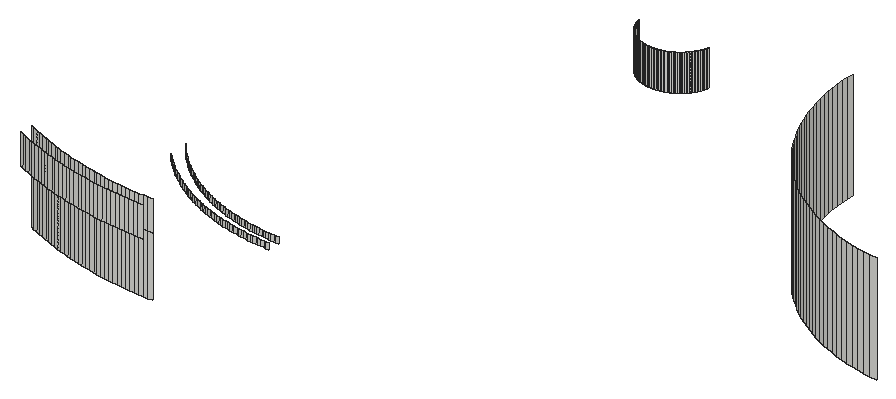
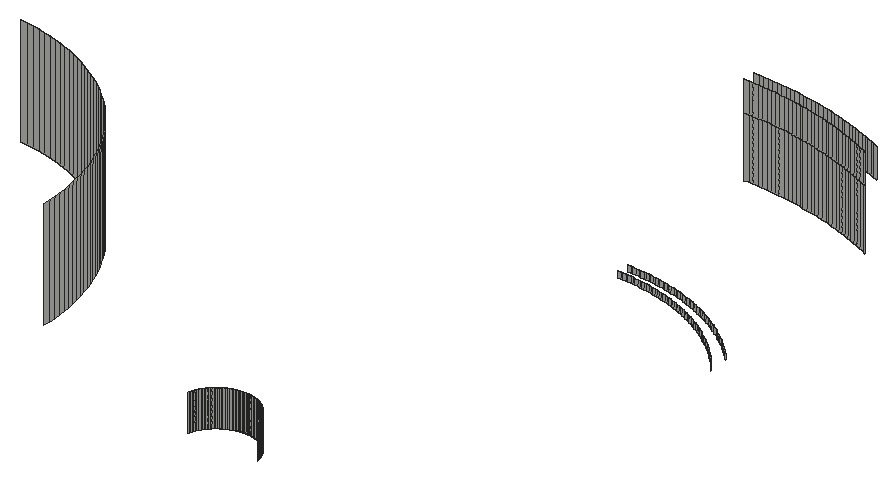
# SketchUp Ruby script. Lengths in inches.
U = 1.inch
M = Sketchup.active_model
def pt(a) = Geom::Point3d.new(a.map { |v| v * U })
def face(e, loops, mat)
  f = e.add_face(loops[0].map { |a| pt(a) })
  loops[1..].each { |l| e.add_face(l.map { |a| pt(a) }).erase! }
  f.material = f.back_material = mat if mat
  f
end
# faces: each face lists its corners as indices into pts; further lists are holes
def faces(e, pts, list, mat = nil) = list.each { |f| face(e, (f[0].is_a?(Array) ? f : [f]).map { |l| l.map { |i| pts[i] } }, mat) }
# xy, xz, yz: faces in a plane at the given z, y or x. An outline is a flat list of corners, or four numbers for a rectangle; further outlines are holes
def ring(l) = l.size == 4 ? [[l[0], l[1]], [l[2], l[1]], [l[2], l[3]], [l[0], l[3]]] : l.each_slice(2).to_a
def flat(e, list, mat, &to3) = list.each { |f| face(e, (f[0].is_a?(Array) ? f : [f]).map { |l| ring(l).map { |u, v| to3.(u, v) } }, mat) }
def xy(e, z, list, mat = nil) = flat(e, list, mat) { |x, y| [x, y, z] }
def xz(e, y, list, mat = nil) = flat(e, list, mat) { |x, z| [x, y, z] }
def yz(e, x, list, mat = nil) = flat(e, list, mat) { |y, z| [x, y, z] }
def lines(e, pts, list) = list.each { |a, b| e.add_line(pt(pts[a]), pt(pts[b])) }
# prism: a flat outline (further loops are holes) pulled along v
def prism(e, loops, v, mat = nil)
  f = face(e, loops, mat); d = Geom::Vector3d.new(v.map { |x| x * U })
  f.pushpull(f.normal.samedirection?(d) ? d.length : -d.length)
end
def box(e, o, s, mat = nil) = prism(e, [[o, [o[0] + s[0], o[1], o[2]], [o[0] + s[0], o[1] + s[1], o[2]], [o[0], o[1] + s[1], o[2]]]], [0, 0, s[2]], mat)
def at(x, y, z, deg = 0) = Geom::Transformation.translation(pt([x, y, z])) * Geom::Transformation.rotation(ORIGIN, Z_AXIS, deg.degrees)
def axes(o, x, y, z) = Geom::Transformation.new([*x, 0, *y, 0, *z, 0, *pt(o).to_a, 1])
def part(name) = M.definitions.add(name)
# library, detail: a bought-in or finely detailed component or shape, given as its bounding box
def library(name, o, s) = part(name).tap { |d| box(d.entities, o, s) }
def detail(e, o, s) = box(e.add_group.entities, o, s)
def put(e, d, t, mat = nil) = e.add_instance(d, t).tap { |i| i.material = mat if mat }
def group(e, t, mat = nil) = e.add_group.tap { |g| g.transformation = t; g.material = mat if mat }.entities
root = M.entities
xz(root,204,[[38.61,354.5,39,357]])
xz(root,205,[[38.62,349.5,39,354.5],[38.62,354.5,39,357]])
xz(root,217,[[38.78,348,39,348.5]])
xz(root,217.01,[[38.33,348,38.55,348.5]])
xz(root,218,[[38.79,348,39,348.5]])
xz(root,218.01,[[38.37,348,38.58,348.5]])
xz(root,249,[[44.84,348,44.92,351],[44.92,348,45,351],[45,348,45.08,351],[45.08,348,45.16,351]])
p = [[37.89,217.04,348],[37.67,217.05,348],[37.67,217.05,348.5],[37.89,217.04,348.5],[38.11,217.02,348],[38.11,217.02,348.5],
  [38.33,217.01,348],[38.33,217.01,348.5],[38.78,217,348],[38.55,217.01,348],[38.55,217.01,348.5],[38.78,217,348.5],
  [36.78,217.15,348],[36.5625,217.18,348],[36.5625,217.18,348.5],[36.78,217.15,348.5],[37,217.12,348],[37,217.12,348.5],
  [37.22,217.09,348],[37.22,217.09,348.5],[37.44,217.07,348],[37.44,217.07,348.5],[36.12,217.25,348],[35.9,217.28,348],
  [35.9,217.28,348.5],[36.12,217.25,348.5],[36.34,217.21,348],[36.34,217.21,348.5],[35.68,217.33,348],[35.47,217.37,348],
  [35.47,217.37,348.5],[35.68,217.33,348.5],[35.25,217.42,348],[35.03,217.47,348],[35.03,217.47,348.5],[35.25,217.42,348.5],
  [34.82,217.52,348],[34.6,217.58,348],[34.6,217.58,348.5],[34.82,217.52,348.5],[34.39,217.64,348],[34.17,217.7,348],
  [34.17,217.7,348.5],[34.39,217.64,348.5],[33.96,217.76,348],[33.96,217.76,348.5],[33.75,217.83,348],[33.54,217.9,348],
  [33.54,217.9,348.5],[33.75,217.83,348.5],[33.33,217.98,348],[33.33,217.98,348.5],[33.12,218.05,348],[33.12,218.05,348.5],
  [37.54,218.07,348],[37.74,218.05,348],[37.74,218.05,348.5],[37.54,218.07,348.5],[37.95,218.03,348],[37.95,218.03,348.5],
  [38.16,218.02,348],[38.16,218.02,348.5],[38.37,218.01,348],[38.37,218.01,348.5],[38.58,218.01,348],[38.79,218,348],
  [38.79,218,348.5],[38.58,218.01,348.5],[32.91,218.13,348],[32.7,218.21,348],[32.7,218.21,348.5],[32.91,218.13,348.5],
  [36.7,218.17,348],[36.91,218.14,348],[36.91,218.14,348.5],[36.7,218.17,348.5],[37.12,218.11,348],[37.12,218.11,348.5],
  [37.33,218.09,348],[37.33,218.09,348.5],[32.49,218.29,348],[32.49,218.29,348.5],[36.08,218.27,348],[36.29,218.23,348],
  [36.29,218.23,348.5],[36.08,218.27,348.5],[36.5,218.2,348],[36.5,218.2,348.5],[32.29,218.38,348],[32.29,218.38,348.5],
  [35.47,218.39,348],[35.67,218.35,348],[35.67,218.35,348.5],[35.47,218.39,348.5],[35.88,218.31,348],[35.88,218.31,348.5],
  [32.09,218.47,348],[32.09,218.47,348.5],[35.0625,218.49,348],[35.26,218.44,348],[35.26,218.44,348.5],[35.0625,218.49,348.5],
  [31.88,218.5625,348],[31.88,218.5625,348.5],[34.66,218.6,348],[34.86,218.55,348],[34.86,218.55,348.5],[34.66,218.6,348.5],
  [31.68,218.66,348],[31.68,218.66,348.5],[34.46,218.66,348],[34.46,218.66,348.5],[31.48,218.75,348],[31.48,218.75,348.5],
  [34.06,218.78,348],[34.26,218.72,348],[34.26,218.72,348.5],[34.06,218.78,348.5],[31.28,218.85,348],[31.28,218.85,348.5],
  [33.66,218.92,348],[33.86,218.85,348],[33.86,218.85,348.5],[33.66,218.92,348.5],[31.08,218.96,348],[31.08,218.96,348.5],
  [33.46,218.99,348],[33.46,218.99,348.5],[30.89,219.06,348],[30.89,219.06,348.5],[33.27,219.0625,348],[33.27,219.0625,348.5],
  [30.69,219.17,348],[30.69,219.17,348.5],[32.88,219.22,348],[33.07,219.14,348],[33.07,219.14,348.5],[32.88,219.22,348.5],
  [30.5,219.28,348],[30.5,219.28,348.5],[32.68,219.3,348],[32.68,219.3,348.5],[30.31,219.39,348],[30.31,219.39,348.5],
  [32.49,219.38,348],[32.49,219.38,348.5],[30.12,219.51,348],[30.12,219.51,348.5],[32.3,219.47,348],[32.3,219.47,348.5],
  [29.93,219.62,348],[29.93,219.62,348.5],[32.11,219.56,348],[32.11,219.56,348.5],[29.74,219.74,348],[29.74,219.74,348.5],
  [31.92,219.65,348],[31.92,219.65,348.5],[29.56,219.87,348],[29.56,219.87,348.5],[31.55,219.84,348],[31.74,219.74,348],
  [31.74,219.74,348.5],[31.55,219.84,348.5],[31.37,219.9375,348],[31.37,219.9375,348.5],[29.37,219.99,348],[29.37,219.99,348.5],
  [31.18,220.04,348],[31.18,220.04,348.5],[29.1875,220.12,348],[29.1875,220.12,348.5],[31,220.14,348],[31,220.14,348.5],
  [29.01,220.25,348],[29.01,220.25,348.5],[30.82,220.25,348],[30.82,220.25,348.5],[28.83,220.38,348],[28.83,220.38,348.5],
  [30.64,220.36,348],[30.64,220.36,348.5],[28.65,220.51,348],[28.65,220.51,348.5],[30.46,220.47,348],[30.46,220.47,348.5],
  [28.48,220.65,348],[28.48,220.65,348.5],[30.29,220.58,348],[30.29,220.58,348.5],[28.3,220.79,348],[28.3,220.79,348.5],
  [30.11,220.7,348],[30.11,220.7,348.5],[29.9375,220.8125,348],[29.9375,220.8125,348.5],[28.13,220.93,348],[28.13,220.93,348.5],
  [29.77,220.93,348],[29.77,220.93,348.5],[27.96,221.07,348],[27.96,221.07,348.5],[29.6,221.06,348],[29.6,221.06,348.5],
  [27.79,221.22,348],[27.79,221.22,348.5],[29.43,221.18,348],[29.43,221.18,348.5],[27.625,221.37,348],[27.625,221.37,348.5],
  [29.26,221.31,348],[29.26,221.31,348.5],[29.09,221.43,348],[29.09,221.43,348.5],[27.46,221.52,348],[27.46,221.52,348.5],
  [28.93,221.57,348],[28.93,221.57,348.5],[27.3,221.67,348],[27.3,221.67,348.5],[28.77,221.7,348],[28.77,221.7,348.5],
  [27.14,221.82,348],[27.14,221.82,348.5],[28.61,221.83,348],[28.61,221.83,348.5],[26.98,221.98,348],[26.98,221.98,348.5],
  [28.45,221.97,348],[28.45,221.97,348.5],[26.82,222.14,348],[26.82,222.14,348.5],[28.29,222.11,348],[28.29,222.11,348.5],
  [28.14,222.25,348],[28.14,222.25,348.5],[27.99,222.39,348],[27.99,222.39,348.5],[27.84,222.54,348],[27.84,222.54,348.5],
  [27.6875,222.6875,348],[27.6875,222.6875,348.5],[27.54,222.84,348],[27.54,222.84,348.5],[27.39,222.99,348],[27.39,222.99,348.5],
  [27.25,223.14,348],[27.25,223.14,348.5],[27.11,223.29,348],[27.11,223.29,348.5],[26.97,223.45,348],[26.97,223.45,348.5],
  [26.83,223.61,348],[26.83,223.61,348.5],[26.7,223.77,348],[26.7,223.77,348.5],[79.18,228.22,357],[79.74,228.14,357],
  [79.74,228.14,348],[79.18,228.22,348],[80.31,228.08,357],[80.31,228.08,348],[78.63,228.32,357],[78.63,228.32,348],
  [78.07,228.43,357],[78.07,228.43,348],[77.52,228.57,357],[77.52,228.57,348],[76.98,228.71,357],[76.98,228.71,348],
  [76.4375,228.88,357],[76.4375,228.88,348],[75.9,229.0625,357],[75.9,229.0625,348],[75.375,229.26,357],[75.375,229.26,348],
  [74.85,229.48,357],[74.85,229.48,348],[74.34,229.71,357],[74.34,229.71,348],[73.83,229.96,357],[73.83,229.96,348],
  [73.33,230.23,357],[73.33,230.23,348],[72.84,230.51,357],[72.84,230.51,348],[72.36,230.8,357],[72.36,230.8,348],
  [71.88,231.11,357],[71.88,231.11,348],[71.42,231.4375,357],[71.42,231.4375,348],[70.97,231.78,357],[70.97,231.78,348],
  [70.53,232.13,357],[70.53,232.13,348],[70.1,232.5,357],[70.1,232.5,348],[69.68,232.88,357],[69.68,232.88,348],
  [69.27,233.27,357],[69.27,233.27,348],[68.88,233.68,357],[68.88,233.68,348],[68.5,234.1,357],[68.5,234.1,348],
  [68.13,234.53,357],[68.13,234.53,348],[67.78,234.97,357],[67.78,234.97,348],[67.4375,235.42,357],[67.4375,235.42,348],
  [67.11,235.88,357],[67.11,235.88,348],[66.8,236.36,357],[66.8,236.36,348],[66.51,236.84,357],[66.51,236.84,348],
  [66.23,237.33,357],[66.23,237.33,348],[65.96,237.83,357],[65.96,237.83,348],[65.71,238.34,357],[65.71,238.34,348],
  [65.48,238.85,357],[65.48,238.85,348],[65.26,239.375,357],[65.26,239.375,348],[65.0625,239.9,357],[65.0625,239.9,348],
  [64.88,240.4375,357],[64.88,240.4375,348],[64.71,240.98,357],[64.71,240.98,348],[64.57,241.52,357],[64.57,241.52,348],
  [64.43,242.07,357],[64.43,242.07,348],[64.32,242.63,357],[64.32,242.63,348],[64.22,243.18,357],[64.22,243.18,348],
  [64.14,243.74,357],[64.14,243.74,348],[64.08,244.31,357],[64.08,244.31,348],[64.04,244.87,357],[64.04,244.87,348],
  [64.01,245.43,357],[64.01,245.43,348],[64,246,357],[64,246,348],[44.53,249.04,348],[44.45,249.05,348],
  [44.45,249.05,351],[44.53,249.04,351],[44.61,249.03,348],[44.61,249.03,351],[44.6875,249.02,348],[44.6875,249.02,351],
  [44.76,249.01,348],[44.76,249.01,351],[44.84,249,348],[44.84,249,351],[45.24,249.01,348],[45.16,249,348],
  [45.16,249,351],[45.24,249.01,351],[45.3125,249.02,348],[45.3125,249.02,351],[45.39,249.03,348],[45.39,249.03,351],
  [45.47,249.04,348],[45.47,249.04,351],[45.55,249.05,348],[45.55,249.05,351],[44.07,249.15,348],[44,249.17,348],
  [44,249.17,351],[44.07,249.15,351],[44.15,249.125,348],[44.15,249.125,351],[44.22,249.1,348],[44.22,249.1,351],
  [44.3,249.08,348],[44.3,249.08,351],[44.375,249.07,348],[44.375,249.07,351],[45.625,249.07,348],[45.625,249.07,351],
  [45.7,249.08,348],[45.7,249.08,351],[45.78,249.1,348],[45.78,249.1,351],[45.85,249.125,348],[45.85,249.125,351],
  [45.93,249.15,348],[45.93,249.15,351],[46,249.17,348],[46,249.17,351],[43.85,249.23,348],[43.78,249.26,348],
  [43.78,249.26,351],[43.85,249.23,351],[43.92,249.2,348],[43.92,249.2,351],[46.07,249.2,348],[46.07,249.2,351],
  [46.15,249.23,348],[46.15,249.23,351],[46.22,249.26,348],[46.22,249.26,351],[43.64,249.33,348],[43.57,249.36,348],
  [43.57,249.36,351],[43.64,249.33,351],[43.71,249.29,348],[43.71,249.29,351],[46.29,249.29,348],[46.29,249.29,351],
  [46.36,249.33,348],[46.36,249.33,351],[46.43,249.36,348],[46.43,249.36,351],[43.43,249.44,348],[43.37,249.48,348],
  [43.37,249.48,351],[43.43,249.44,351],[43.5,249.4,348],[43.5,249.4,351],[46.5,249.4,348],[46.5,249.4,351],
  [46.57,249.44,348],[46.57,249.44,351],[46.63,249.48,348],[46.63,249.48,351],[43.3,249.53,348],[43.24,249.57,348],
  [43.24,249.57,351],[43.3,249.53,351],[46.7,249.53,348],[46.7,249.53,351],[46.76,249.57,348],[46.76,249.57,351],
  [43.17,249.62,348],[43.11,249.67,348],[43.11,249.67,351],[43.17,249.62,351],[46.83,249.62,348],[46.83,249.62,351],
  [46.89,249.67,348],[46.89,249.67,351],[43.05,249.72,348],[42.99,249.77,348],[42.99,249.77,351],[43.05,249.72,351],
  [46.95,249.72,348],[46.95,249.72,351],[47.01,249.77,348],[47.01,249.77,351],[42.93,249.82,348],[42.88,249.88,348],
  [42.88,249.88,351],[42.93,249.82,351],[47.06,249.82,348],[47.06,249.82,351],[47.12,249.88,348],[47.12,249.88,351],
  [42.82,249.94,348],[42.77,249.99,348],[42.77,249.99,351],[42.82,249.94,351],[47.18,249.93,348],[47.18,249.93,351],
  [47.23,249.99,348],[47.23,249.99,351],[42.72,250.05,348],[42.72,250.05,351],[47.28,250.05,348],[47.28,250.05,351],
  [42.67,250.11,348],[42.62,250.17,348],[42.62,250.17,351],[42.67,250.11,351],[47.33,250.11,348],[47.33,250.11,351],
  [47.38,250.17,348],[47.38,250.17,351],[42.57,250.24,348],[42.53,250.3,348],[42.53,250.3,351],[42.57,250.24,351],
  [47.43,250.24,348],[47.43,250.24,351],[47.47,250.3,348],[47.47,250.3,351],[42.48,250.37,348],[42.48,250.37,351],
  [47.52,250.37,348],[47.52,250.37,351],[42.44,250.43,348],[42.4,250.5,348],[42.4,250.5,351],[42.44,250.43,351],
  [47.56,250.43,348],[47.56,250.43,351],[47.6,250.5,348],[47.6,250.5,351],[42.36,250.57,348],[42.36,250.57,351],
  [47.64,250.57,348],[47.64,250.57,351],[42.33,250.64,348],[42.29,250.71,348],[42.29,250.71,351],[42.33,250.64,351],
  [47.67,250.64,348],[47.67,250.64,351],[47.71,250.71,348],[47.71,250.71,351],[42.26,250.78,348],[42.26,250.78,351],
  [47.74,250.78,348],[47.74,250.78,351],[42.23,250.85,348],[42.23,250.85,351],[47.77,250.85,348],[47.77,250.85,351],
  [42.2,250.93,348],[42.17,251,348],[42.17,251,351],[42.2,250.93,351],[47.8,250.92,348],[47.8,250.92,351],
  [47.83,251,348],[47.83,251,351],[42.15,251.07,348],[42.15,251.07,351],[47.85,251.07,348],[47.85,251.07,351],
  [42.125,251.15,348],[42.1,251.22,348],[42.1,251.22,351],[42.125,251.15,351],[47.875,251.15,348],[47.875,251.15,351],
  [47.9,251.22,348],[47.9,251.22,351],[42.08,251.3,348],[42.08,251.3,351],[47.92,251.3,348],[47.92,251.3,351],
  [37.1,205.0625,349.5],[37.48,205.04,349.5],[37.48,205.04,354.5],[37.1,205.0625,354.5],[37.86,205.02,349.5],[37.86,205.02,354.5],
  [38.24,205.01,349.5],[38.24,205.01,354.5],[38.62,205,349.5],[38.62,205,354.5],[35.97,205.16,349.5],[36.35,205.12,349.5],
  [36.35,205.12,354.5],[35.97,205.16,354.5],[36.72,205.09,349.5],[36.72,205.09,354.5],[34.84,205.3,349.5],[35.21,205.25,349.5],
  [35.21,205.25,354.5],[34.84,205.3,354.5],[35.59,205.2,349.5],[35.59,205.2,354.5],[34.46,205.36,349.5],[34.46,205.36,354.5],
  [33.72,205.49,349.5],[34.09,205.42,349.5],[34.09,205.42,354.5],[33.72,205.49,354.5],[33.34,205.56,349.5],[33.34,205.56,354.5],
  [32.6,205.72,349.5],[32.97,205.63,349.5],[32.97,205.63,354.5],[32.6,205.72,354.5],[32.23,205.8,349.5],[32.23,205.8,354.5],
  [31.86,205.89,349.5],[31.86,205.89,354.5],[31.49,205.99,349.5],[31.49,205.99,354.5],[31.13,206.09,349.5],[31.13,206.09,354.5],
  [30.76,206.19,349.5],[30.76,206.19,354.5],[30.4,206.3,349.5],[30.4,206.3,354.5],[30.04,206.42,349.5],[30.04,206.42,354.5],
  [29.68,206.54,349.5],[29.68,206.54,354.5],[29.32,206.66,349.5],[29.32,206.66,354.5],[28.96,206.79,349.5],[28.96,206.79,354.5],
  [28.61,206.93,349.5],[28.61,206.93,354.5],[28.25,207.06,349.5],[28.25,207.06,354.5],[27.9,207.21,349.5],[27.9,207.21,354.5],
  [27.55,207.36,349.5],[27.55,207.36,354.5],[27.2,207.51,349.5],[27.2,207.51,354.5],[26.86,207.66,349.5],[26.86,207.66,354.5],
  [37.04,204.0625,354.5],[37.43,204.04,354.5],[37.43,204.04,357],[37.04,204.0625,357],[37.82,204.02,354.5],[37.82,204.02,357],
  [38.21,204.01,354.5],[38.21,204.01,357],[38.61,204,354.5],[38.61,204,357],[35.86,204.16,354.5],[36.25,204.125,354.5],
  [36.25,204.125,357],[35.86,204.16,357],[36.65,204.09,354.5],[36.65,204.09,357],[35.08,204.26,354.5],[35.47,204.21,354.5],
  [35.47,204.21,357],[35.08,204.26,357],[34.31,204.37,354.5],[34.7,204.31,354.5],[34.7,204.31,357],[34.31,204.37,357],
  [33.53,204.5,354.5],[33.92,204.43,354.5],[33.92,204.43,357],[33.53,204.5,357],[33.15,204.58,354.5],[33.15,204.58,357],
  [32.76,204.66,354.5],[32.76,204.66,357],[32,204.83,354.5],[32.38,204.74,354.5],[32.38,204.74,357],[32,204.83,357],
  [31.62,204.92,354.5],[31.62,204.92,357],[31.24,205.02,354.5],[31.24,205.02,357],[30.86,205.125,354.5],[30.86,205.125,357],
  [37.1,205.0625,357],[37.48,205.04,357],[37.86,205.02,357],[38.24,205.01,357],[38.62,205,357],[30.48,205.24,354.5],
  [30.48,205.24,357],[35.97,205.16,357],[36.35,205.12,357],[36.72,205.09,357],[30.1,205.35,354.5],[30.1,205.35,357],
  [34.84,205.3,357],[35.21,205.25,357],[35.59,205.2,357],[29.73,205.47,354.5],[29.73,205.47,357],[34.46,205.36,357],
  [33.72,205.49,357],[34.09,205.42,357],[29.36,205.59,354.5],[29.36,205.59,357],[33.34,205.56,357],[28.99,205.72,354.5],
  [28.99,205.72,357],[32.6,205.72,357],[32.97,205.63,357],[28.62,205.85,354.5],[28.62,205.85,357],[32.23,205.8,357],
  [31.86,205.89,357],[28.25,205.99,354.5],[28.25,205.99,357],[31.49,205.99,357],[27.88,206.14,354.5],[27.88,206.14,357],
  [31.13,206.09,357],[27.52,206.28,354.5],[27.52,206.28,357],[30.76,206.19,357],[30.4,206.3,357],[27.16,206.4375,354.5],
  [27.16,206.4375,357],[30.04,206.42,357],[26.8,206.59,354.5],[26.8,206.59,357],[29.68,206.54,357],[29.32,206.66,357],
  [28.96,206.79,357],[28.61,206.93,357],[28.25,207.06,357],[27.9,207.21,357],[27.55,207.36,357],[27.2,207.51,357],
  [26.86,207.66,357]]
faces(root,p,[[0,1,2,3],[4,0,3,5],[6,4,5,7],[8,9,10,11],[12,13,14,15],[16,12,15,17],[18,16,17,19],[20,18,19,21],
  [1,20,21,2],[22,23,24,25],[26,22,25,27],[13,26,27,14],[28,29,30,31],[23,28,31,24],[32,33,34,35],[29,32,35,30],
  [36,37,38,39],[33,36,39,34],[40,41,42,43],[37,40,43,38],[41,44,45,42],[46,47,48,49],[44,46,49,45],[47,50,51,48],
  [50,52,53,51],[54,55,56,57],[55,58,59,56],[58,60,61,59],[60,62,63,61],[64,65,66,67],[68,69,70,71],[52,68,71,53],
  [72,73,74,75],[73,76,77,74],[76,78,79,77],[78,54,57,79],[69,80,81,70],[82,83,84,85],[83,86,87,84],[86,72,75,87],
  [80,88,89,81],[90,91,92,93],[91,94,95,92],[94,82,85,95],[88,96,97,89],[98,99,100,101],[99,90,93,100],[96,102,103,97],
  [104,105,106,107],[105,98,101,106],[102,108,109,103],[110,104,107,111],[108,112,113,109],[114,115,116,117],[115,110,111,116],[112,118,119,113],
  [120,121,122,123],[121,114,117,122],[118,124,125,119],[126,120,123,127],[124,128,129,125],[130,126,127,131],[128,132,133,129],[134,135,136,137],
  [135,130,131,136],[132,138,139,133],[140,134,137,141],[138,142,143,139],[144,140,141,145],[142,146,147,143],[148,144,145,149],[146,150,151,147],
  [152,148,149,153],[150,154,155,151],[156,152,153,157],[154,158,159,155],[160,161,162,163],[161,156,157,162],[164,160,163,165],[158,166,167,159],
  [168,164,165,169],[166,170,171,167],[172,168,169,173],[170,174,175,171],[176,172,173,177],[174,178,179,175],[180,176,177,181],[178,182,183,179],
  [184,180,181,185],[182,186,187,183],[188,184,185,189],[186,190,191,187],[192,188,189,193],[194,192,193,195],[190,196,197,191],[198,194,195,199],
  [196,200,201,197],[202,198,199,203],[200,204,205,201],[206,202,203,207],[204,208,209,205],[210,206,207,211],[212,210,211,213],[208,214,215,209],
  [216,212,213,217],[214,218,219,215],[220,216,217,221],[218,222,223,219],[224,220,221,225],[222,226,227,223],[228,224,225,229],[226,230,231,227],
  [232,228,229,233],[234,232,233,235],[236,234,235,237],[238,236,237,239],[240,238,239,241],[242,240,241,243],[244,242,243,245],[246,244,245,247],
  [248,246,247,249],[250,248,249,251],[252,250,251,253],[254,252,253,255],[256,257,258,259],[257,260,261,258],[262,256,259,263],[264,262,263,265],
  [266,264,265,267],[268,266,267,269],[270,268,269,271],[272,270,271,273],[274,272,273,275],[276,274,275,277],[278,276,277,279],[280,278,279,281],
  [282,280,281,283],[284,282,283,285],[286,284,285,287],[288,286,287,289],[290,288,289,291],[292,290,291,293],[294,292,293,295],[296,294,295,297],
  [298,296,297,299],[300,298,299,301],[302,300,301,303],[304,302,303,305],[306,304,305,307],[308,306,307,309],[310,308,309,311],[312,310,311,313],
  [314,312,313,315],[316,314,315,317],[318,316,317,319],[320,318,319,321],[322,320,321,323],[324,322,323,325],[326,324,325,327],[328,326,327,329],
  [330,328,329,331],[332,330,331,333],[334,332,333,335],[336,334,335,337],[338,336,337,339],[340,338,339,341],[342,340,341,343],[344,342,343,345],
  [346,344,345,347],[348,346,347,349],[350,348,349,351],[352,353,354,355],[356,352,355,357],[358,356,357,359],[360,358,359,361],[362,360,361,363],
  [364,365,366,367],[368,364,367,369],[370,368,369,371],[372,370,371,373],[374,372,373,375],[376,377,378,379],[380,376,379,381],[382,380,381,383],
  [384,382,383,385],[386,384,385,387],[353,386,387,354],[388,374,375,389],[390,388,389,391],[392,390,391,393],[394,392,393,395],[396,394,395,397],
  [398,396,397,399],[400,401,402,403],[404,400,403,405],[377,404,405,378],[406,398,399,407],[408,406,407,409],[410,408,409,411],[412,413,414,415],
  [416,412,415,417],[401,416,417,402],[418,410,411,419],[420,418,419,421],[422,420,421,423],[424,425,426,427],[428,424,427,429],[413,428,429,414],
  [430,422,423,431],[432,430,431,433],[434,432,433,435],[436,437,438,439],[425,436,439,426],[440,434,435,441],[442,440,441,443],[444,445,446,447],
  [437,444,447,438],[448,442,443,449],[450,448,449,451],[452,453,454,455],[445,452,455,446],[456,450,451,457],[458,456,457,459],[460,461,462,463],
  [453,460,463,454],[464,458,459,465],[466,464,465,467],[468,469,470,471],[461,468,471,462],[472,466,467,473],[474,472,473,475],[469,476,477,470],
  [478,474,475,479],[480,481,482,483],[476,480,483,477],[484,478,479,485],[486,484,485,487],[488,489,490,491],[481,488,491,482],[492,486,487,493],
  [494,492,493,495],[489,496,497,490],[498,494,495,499],[500,501,502,503],[496,500,503,497],[504,498,499,505],[506,504,505,507],[501,508,509,502],
  [510,506,507,511],[512,513,514,515],[508,512,515,509],[516,510,511,517],[518,516,517,519],[513,520,521,514],[522,518,519,523],[520,524,525,521],
  [526,522,523,527],[528,529,530,531],[524,528,531,525],[532,526,527,533],[534,532,533,535],[529,536,537,530],[538,534,535,539],[540,541,542,543],
  [536,540,543,537],[544,538,539,545],[546,544,545,547],[541,548,549,542],[550,546,547,551],[552,553,554,555],[553,556,557,554],[556,558,559,557],
  [558,560,561,559],[562,563,564,565],[563,566,567,564],[566,552,555,567],[568,569,570,571],[569,572,573,570],[572,562,565,573],[574,568,571,575],
  [576,577,578,579],[577,574,575,578],[580,576,579,581],[582,583,584,585],[583,580,581,584],[586,582,585,587],[588,586,587,589],[590,588,589,591],
  [592,590,591,593],[594,592,593,595],[596,594,595,597],[598,596,597,599],[600,598,599,601],[602,600,601,603],[604,602,603,605],[606,604,605,607],
  [608,606,607,609],[610,608,609,611],[612,610,611,613],[614,612,613,615],[616,614,615,617],[618,619,620,621],[619,622,623,620],[622,624,625,623],
  [624,626,627,625],[628,629,630,631],[629,632,633,630],[632,618,621,633],[634,635,636,637],[635,628,631,636],[638,639,640,641],[639,634,637,640],
  [642,643,644,645],[643,638,641,644],[646,642,645,647],[648,646,647,649],[650,651,652,653],[651,648,649,652],[654,650,653,655],[656,654,655,657],
  [658,656,657,659],[554,555,660,661],[557,554,661,662],[559,557,662,663],[561,559,663,664],[665,658,659,666],[564,565,667,668],[567,564,668,669],
  [555,567,669,660],[670,665,666,671],[570,571,672,673],[573,570,673,674],[565,573,674,667],[675,670,671,676],[571,575,677,672],[578,579,678,679],
  [575,578,679,677],[680,675,676,681],[579,581,682,678],[683,680,681,684],[584,585,685,686],[581,584,686,682],[687,683,684,688],[585,587,689,685],
  [587,589,690,689],[691,687,688,692],[589,591,693,690],[694,691,692,695],[591,593,696,693],[697,694,695,698],[593,595,699,696],[595,597,700,699],
  [701,697,698,702],[597,599,703,700],[704,701,702,705],[599,601,706,703],[601,603,707,706],[603,605,708,707],[605,607,709,708],[607,609,710,709],
  [609,611,711,710],[611,613,712,711],[613,615,713,712],[615,617,714,713]])
